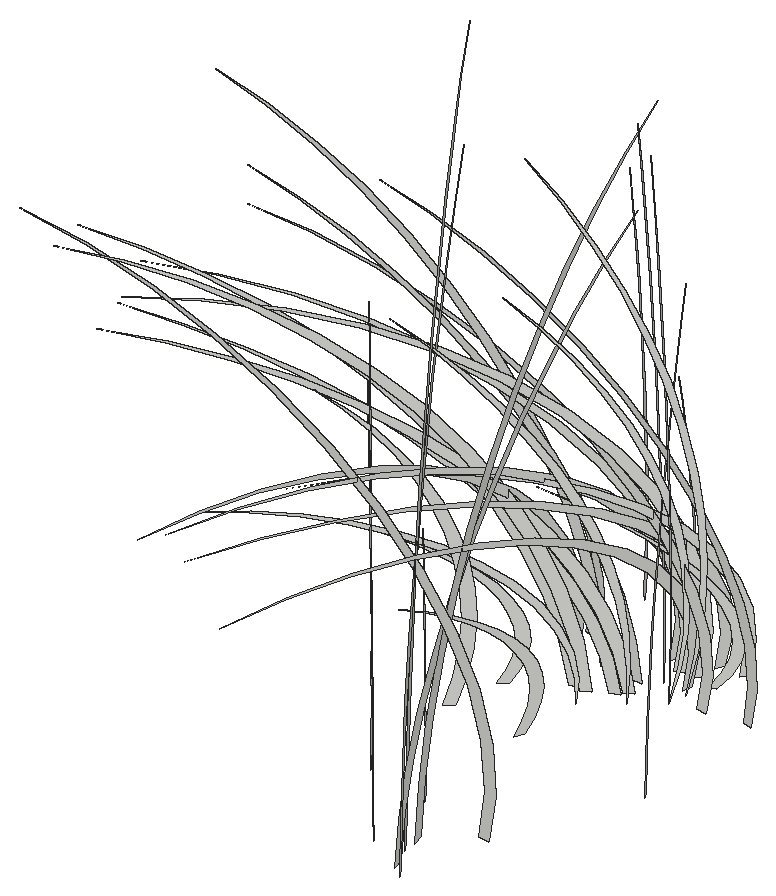
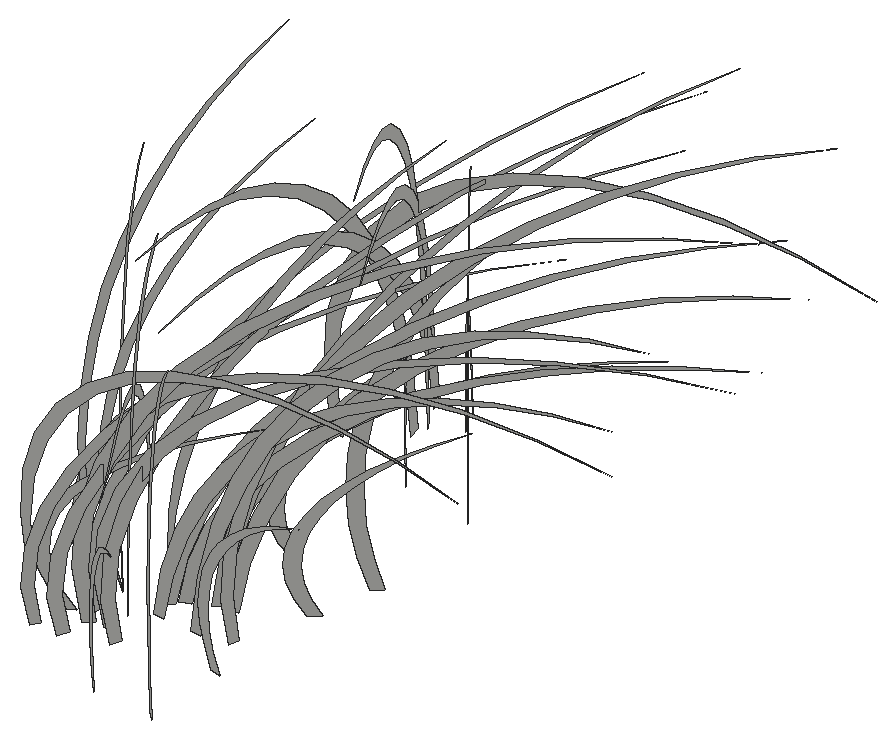
# SketchUp Ruby script. Lengths in inches.
U = 1.inch
M = Sketchup.active_model
def pt(a) = Geom::Point3d.new(a.map { |v| v * U })
def face(e, loops, mat)
  f = e.add_face(loops[0].map { |a| pt(a) })
  loops[1..].each { |l| e.add_face(l.map { |a| pt(a) }).erase! }
  f.material = f.back_material = mat if mat
  f
end
# faces: each face lists its corners as indices into pts; further lists are holes
def faces(e, pts, list, mat = nil) = list.each { |f| face(e, (f[0].is_a?(Array) ? f : [f]).map { |l| l.map { |i| pts[i] } }, mat) }
# xy, xz, yz: faces in a plane at the given z, y or x. An outline is a flat list of corners, or four numbers for a rectangle; further outlines are holes
def ring(l) = l.size == 4 ? [[l[0], l[1]], [l[2], l[1]], [l[2], l[3]], [l[0], l[3]]] : l.each_slice(2).to_a
def flat(e, list, mat, &to3) = list.each { |f| face(e, (f[0].is_a?(Array) ? f : [f]).map { |l| ring(l).map { |u, v| to3.(u, v) } }, mat) }
def xy(e, z, list, mat = nil) = flat(e, list, mat) { |x, y| [x, y, z] }
def xz(e, y, list, mat = nil) = flat(e, list, mat) { |x, z| [x, y, z] }
def yz(e, x, list, mat = nil) = flat(e, list, mat) { |y, z| [x, y, z] }
def lines(e, pts, list) = list.each { |a, b| e.add_line(pt(pts[a]), pt(pts[b])) }
# prism: a flat outline (further loops are holes) pulled along v
def prism(e, loops, v, mat = nil)
  f = face(e, loops, mat); d = Geom::Vector3d.new(v.map { |x| x * U })
  f.pushpull(f.normal.samedirection?(d) ? d.length : -d.length)
end
def box(e, o, s, mat = nil) = prism(e, [[o, [o[0] + s[0], o[1], o[2]], [o[0] + s[0], o[1] + s[1], o[2]], [o[0], o[1] + s[1], o[2]]]], [0, 0, s[2]], mat)
def at(x, y, z, deg = 0) = Geom::Transformation.translation(pt([x, y, z])) * Geom::Transformation.rotation(ORIGIN, Z_AXIS, deg.degrees)
def axes(o, x, y, z) = Geom::Transformation.new([*x, 0, *y, 0, *z, 0, *pt(o).to_a, 1])
def part(name) = M.definitions.add(name)
# library, detail: a bought-in or finely detailed component or shape, given as its bounding box
def library(name, o, s) = part(name).tap { |d| box(d.entities, o, s) }
def detail(e, o, s) = box(e.add_group.entities, o, s)
def put(e, d, t, mat = nil) = e.add_instance(d, t).tap { |i| i.material = mat if mat }
def group(e, t, mat = nil) = e.add_group.tap { |g| g.transformation = t; g.material = mat if mat }.entities
root = M.entities
g1 = group(root,at(60.56,581.97,0.02))
p = [[-17.05,1.34,17.08],[-19.62,1.54,17.53],[-17.13,1.35,16.98],[-14.72,1.16,16.23],[-12.43,0.98,15.27],[-10.27,0.81,14.125],
  [-8.28,0.65,12.8],[-6.47,0.51,11.3125],[-4.86,0.38,9.68],[-3.48,0.27,7.92],[-2.34,0.18,6.05],[-1.44,0.11,4.09],
  [-0.81,0.0625,2.07],[-0.44,0.03,0],[0,0,0],[-0.3,0.02,2.11],[-0.89,0.07,4.1875],[-1.77,0.14,6.19],
  [-2.92,0.23,8.11],[-4.34,0.34,9.9],[-5.99,0.47,11.56],[-7.86,0.62,13.05],[-9.93,0.78,14.37],[-12.17,0.96,15.49],
  [-14.55,1.15,16.39]]
faces(g1,p,[[0,1,2,3,4,5,6,7,8,9,10,11,12,13,14,15,16,17,18,19,20,21,22,23,24]])
g2 = group(root,at(60.53,580.25,0.02))
p = [[-16.35,-5,14.86],[-18.82,-5.75,15.25],[-16.43,-5.02,14.77],[-14.12,-4.32,14.12],[-11.92,-3.65,13.29],[-9.85,-3.01,12.29],
  [-7.94,-2.43,11.14],[-6.21,-1.9,9.84],[-4.67,-1.43,8.42],[-3.34,-1.02,6.89],[-2.24,-0.69,5.26],[-1.38,-0.42,3.56],
  [-0.78,-0.24,1.8],[-0.43,-0.13,0],[0,0,0],[-0.29,-0.09,1.84],[-0.86,-0.26,3.64],[-1.7,-0.52,5.39],
  [-2.81,-0.86,7.05],[-4.16,-1.27,8.62],[-5.75,-1.76,10.06],[-7.54,-2.31,11.36],[-9.53,-2.91,12.5],[-11.68,-3.57,13.47],
  [-13.96,-4.27,14.26]]
faces(g2,p,[[0,1,2,3,4,5,6,7,8,9,10,11,12,13,14,15,16,17,18,19,20,21,22,23,24]])
g3 = group(root,at(62.14,581.84,0.02))
p = [[-17.05,1.34,13.77],[-19.62,1.54,14.14],[-17.13,1.35,13.7],[-14.72,1.16,13.09],[-12.43,0.98,12.32],[-10.27,0.81,11.39],
  [-8.28,0.65,10.32],[-6.47,0.51,9.12],[-4.86,0.38,7.8],[-3.48,0.27,6.38],[-2.34,0.18,4.875],[-1.44,0.11,3.3],
  [-0.81,0.0625,1.67],[-0.44,0.03,0],[0,0,0],[-0.3,0.02,1.71],[-0.89,0.07,3.38],[-1.77,0.14,4.99],
  [-2.92,0.23,6.54],[-4.34,0.34,7.99],[-5.99,0.47,9.32],[-7.86,0.62,10.53],[-9.93,0.78,11.59],[-12.17,0.96,12.49],
  [-14.55,1.15,13.22]]
faces(g3,p,[[0,1,2,3,4,5,6,7,8,9,10,11,12,13,14,15,16,17,18,19,20,21,22,23,24]])
g4 = group(root,at(65.52,569.11,0.02))
p = [[-0.91,0.16,0],[-0.4,0.07,0],[0,0,2.0625],[-0.16,0.03,4.13],[-0.89,0.16,6.16],[-2.17,0.39,8.1],
  [-3.95,0.7,9.91],[-6.21,1.11,11.52],[-8.88,1.58,12.92],[-11.91,2.12,14.05],[-15.2,2.71,14.9],[-18.68,3.33,15.45],
  [-22.27,3.97,15.67],[-25.88,4.61,15.5625],[-22.34,3.98,15.58],[-18.84,3.36,15.29],[-15.45,2.75,14.71],[-12.26,2.18,13.83],
  [-9.34,1.66,12.68],[-6.75,1.2,11.3],[-4.56,0.8125,9.7],[-2.81,0.5,7.9375],[-1.55,0.28,6.04],[-0.8,0.14,4.05],
  [-0.59,0.1,2.02]]
faces(g4,p,[[0,1,2,3,4,5,6,7,8,9,10,11,12,13,14,15,16,17,18,19,20,21,22,23,24]])
g5 = group(root,at(65.52,569.11,0.02))
p = [[-0.91,0.16,0],[-0.4,0.07,0],[0,0,2.0625],[-0.16,0.03,4.13],[-0.89,0.16,6.16],[-2.17,0.39,8.1],
  [-3.95,0.7,9.91],[-6.21,1.11,11.52],[-8.88,1.58,12.92],[-11.91,2.12,14.05],[-15.2,2.71,14.9],[-18.68,3.33,15.45],
  [-22.27,3.97,15.67],[-25.88,4.61,15.5625],[-22.34,3.98,15.58],[-18.84,3.36,15.29],[-15.45,2.75,14.71],[-12.26,2.18,13.83],
  [-9.34,1.66,12.68],[-6.75,1.2,11.3],[-4.56,0.8125,9.7],[-2.81,0.5,7.9375],[-1.55,0.28,6.04],[-0.8,0.14,4.05],
  [-0.59,0.1,2.02]]
faces(g5,p,[[0,1,2,3,4,5,6,7,8,9,10,11,12,13,14,15,16,17,18,19,20,21,22,23,24]])
g6 = group(root,at(62.05,580.72,0.02))
p = [[-16.35,-5,11.98],[-18.82,-5.75,12.3],[-16.43,-5.02,11.91],[-14.12,-4.32,11.39],[-11.92,-3.65,10.71],[-9.85,-3.01,9.91],
  [-7.94,-2.43,8.98],[-6.21,-1.9,7.9375],[-4.67,-1.43,6.79],[-3.34,-1.02,5.55],[-2.24,-0.69,4.24],[-1.38,-0.42,2.87],
  [-0.78,-0.24,1.45],[-0.43,-0.13,0],[0,0,0],[-0.29,-0.09,1.48],[-0.86,-0.26,2.9375],[-1.7,-0.52,4.35],
  [-2.81,-0.86,5.6875],[-4.16,-1.27,6.95],[-5.75,-1.76,8.11],[-7.54,-2.31,9.16],[-9.53,-2.91,10.08],[-11.68,-3.57,10.87],
  [-13.96,-4.27,11.5]]
faces(g6,p,[[0,1,2,3,4,5,6,7,8,9,10,11,12,13,14,15,16,17,18,19,20,21,22,23,24]])
g7 = group(root,at(61.05,580.28,0.02))
p = [[-14.34,-9.3125,17.08],[-16.51,-10.72,17.53],[-14.41,-9.36,16.98],[-12.39,-8.04,16.23],[-10.46,-6.79,15.27],[-8.64,-5.61,14.125],
  [-6.96,-4.52,12.8],[-5.44,-3.53,11.3125],[-4.09,-2.66,9.68],[-2.93,-1.9,7.92],[-1.97,-1.28,6.05],[-1.21,-0.79,4.09],
  [-0.68,-0.44,2.07],[-0.375,-0.24,0],[0,0,0],[-0.25,-0.16,2.11],[-0.75,-0.49,4.1875],[-1.49,-0.97,6.19],
  [-2.46,-1.6,8.11],[-3.65,-2.37,9.9],[-5.04,-3.27,11.56],[-6.61,-4.3,13.05],[-8.36,-5.43,14.37],[-10.24,-6.65,15.49],
  [-12.24,-7.95,16.39]]
faces(g7,p,[[0,1,2,3,4,5,6,7,8,9,10,11,12,13,14,15,16,17,18,19,20,21,22,23,24]])
g8 = group(root,at(63.18,583.56,0.02))
p = [[-0.73,-0.22,0],[-0.32,-0.1,0],[0,0,1.7],[-0.13,-0.04,3.4],[-0.71,-0.22,5.07],[-1.73,-0.53,6.67],
  [-3.16,-0.97,8.15],[-4.97,-1.52,9.48],[-7.1,-2.17,10.63],[-9.52,-2.91,11.57],[-12.15,-3.71,12.27],[-14.9375,-4.57,12.71],
  [-17.81,-5.44,12.89],[-20.6875,-6.33,12.81],[-17.86,-5.46,12.82],[-15.0625,-4.6,12.59],[-12.35,-3.78,12.1],[-9.8,-3,11.38],
  [-7.47,-2.28,10.4375],[-5.4,-1.65,9.3],[-3.64,-1.11,7.99],[-2.25,-0.6875,6.53],[-1.24,-0.38,4.97],[-0.64,-0.2,3.33],
  [-0.47,-0.14,1.67]]
faces(g8,p,[[0,1,2,3,4,5,6,7,8,9,10,11,12,13,14,15,16,17,18,19,20,21,22,23,24]])
g9 = group(root,at(65.68,581.57,0.02))
p = [[-0.81,0.0625,0],[-0.36,0.03,0],[0,0,1.66],[-0.15,0.01,3.32],[-0.8,0.0625,4.96],[-1.9375,0.15,6.52],
  [-3.54,0.28,7.97],[-5.56,0.4375,9.27],[-7.95,0.625,10.39],[-10.65,0.84,11.3],[-13.6,1.07,11.98],[-16.72,1.32,12.42],
  [-19.93,1.57,12.6],[-23.15,1.82,12.51],[-19.99,1.57,12.53],[-16.85,1.33,12.3],[-13.83,1.09,11.82],[-10.97,0.86,11.12],
  [-8.35,0.66,10.2],[-6.04,0.48,9.09],[-4.08,0.32,7.8],[-2.51,0.2,6.38],[-1.39,0.11,4.86],[-0.72,0.06,3.26],
  [-0.53,0.04,1.63]]
faces(g9,p,[[0,1,2,3,4,5,6,7,8,9,10,11,12,13,14,15,16,17,18,19,20,21,22,23,24]])
g10 = group(root,at(62.38,581.15,0.02))
p = [[-14.34,-9.3125,13.77],[-16.51,-10.72,14.14],[-14.41,-9.36,13.7],[-12.39,-8.04,13.09],[-10.46,-6.79,12.32],[-8.64,-5.61,11.39],
  [-6.96,-4.52,10.32],[-5.44,-3.53,9.12],[-4.09,-2.66,7.8],[-2.93,-1.9,6.38],[-1.97,-1.28,4.875],[-1.21,-0.79,3.3],
  [-0.68,-0.44,1.67],[-0.375,-0.24,0],[0,0,0],[-0.25,-0.16,1.71],[-0.75,-0.49,3.38],[-1.49,-0.97,4.99],
  [-2.46,-1.6,6.54],[-3.65,-2.37,7.99],[-5.04,-3.27,9.32],[-6.61,-4.3,10.53],[-8.36,-5.43,11.59],[-10.24,-6.65,12.49],
  [-12.24,-7.95,13.22]]
faces(g10,p,[[0,1,2,3,4,5,6,7,8,9,10,11,12,13,14,15,16,17,18,19,20,21,22,23,24]])
g11 = group(root,at(63.88,583.79,0.02))
p = [[-0.64,-0.41,0],[-0.28,-0.18,0],[0,0,1.95],[-0.11,-0.07,3.91],[-0.625,-0.41,5.83],[-1.52,-0.99,7.67],
  [-2.77,-1.8,9.37],[-4.36,-2.83,10.9],[-6.23,-4.05,12.22],[-8.35,-5.42,13.3],[-10.66,-6.92,14.1],[-13.1,-8.51,14.61],
  [-15.62,-10.14,14.82],[-18.14,-11.78,14.72],[-15.66,-10.17,14.74],[-13.21,-8.58,14.47],[-10.83,-7.04,13.91],[-8.6,-5.58,13.08],
  [-6.55,-4.25,12],[-4.73,-3.07,10.6875],[-3.19,-2.07,9.18],[-1.97,-1.28,7.51],[-1.09,-0.7,5.71],[-0.5625,-0.37,3.83],
  [-0.41,-0.27,1.91]]
faces(g11,p,[[0,1,2,3,4,5,6,7,8,9,10,11,12,13,14,15,16,17,18,19,20,21,22,23,24]])
g12 = group(root,at(61.27,579.25,0.02))
p = [[-10.68,-8.77,8.14],[-9.25,-7.59,8.09],[-7.83,-6.43,7.89],[-6.47,-5.32,7.56],[-5.19,-4.26,7.08],[-4,-3.29,6.49],
  [-2.94,-2.42,5.78],[-2.02,-1.66,4.97],[-1.27,-1.04,4.07],[-0.6875,-0.56,3.11],[-0.29,-0.24,2.09],[-0.1,-0.08,1.05],
  [-0.09,-0.08,0],[0,0,1.07],[-0.125,-0.1,2.14],[-0.47,-0.38,3.19],[-1.02,-0.84,4.1875],[-1.77,-1.45,5.11],
  [-2.7,-2.22,5.94],[-3.79,-3.11,6.67],[-5.01,-4.12,7.26],[-6.35,-5.21,7.71],[-7.76,-6.37,8.02],[-9.21,-7.57,8.16]]
faces(g12,p,[[0,1,2,3,4,5,6,7,8,9,10,11,12,13,14,15,16,17,18,19,20,21,22,23]])
g13 = group(root,at(58.4,576.89,0.02))
p = [[-4.57,-3.75,13.1875],[-3.73,-3.06,12.35],[-2.98,-2.45,11.43],[-2.3125,-1.9,10.45],[-1.74,-1.43,9.4],[-1.26,-1.04,8.29],
  [-0.89,-0.73,7.15],[-0.63,-0.52,5.97],[-0.47,-0.39,4.78],[-0.43,-0.35,3.57],[-0.49,-0.41,2.36],[-0.67,-0.55,1.17],
  [-0.96,-0.78,0],[-0.59,-0.48,0],[-0.27,-0.22,1.1875],[-0.07,-0.0625,2.4],[0,0,3.63],[-0.05,-0.04,4.86],
  [-0.22,-0.18,6.08],[-0.52,-0.43,7.27],[-0.93,-0.76,8.42],[-1.46,-1.2,9.52],[-2.09,-1.72,10.5625],[-2.83,-2.32,11.53],
  [-3.65,-3,12.41]]
faces(g13,p,[[0,1,2,3,4,5,6,7,8,9,10,11,12,13,14,15,16,17,18,19,20,21,22,23,24]])
g14 = group(root,at(58.4,576.89,0.02))
p = [[-4.57,-3.75,13.1875],[-3.73,-3.06,12.35],[-2.98,-2.45,11.43],[-2.3125,-1.9,10.45],[-1.74,-1.43,9.4],[-1.26,-1.04,8.29],
  [-0.89,-0.73,7.15],[-0.63,-0.52,5.97],[-0.47,-0.39,4.78],[-0.43,-0.35,3.57],[-0.49,-0.41,2.36],[-0.67,-0.55,1.17],
  [-0.96,-0.78,0],[-0.59,-0.48,0],[-0.27,-0.22,1.1875],[-0.07,-0.0625,2.4],[0,0,3.63],[-0.05,-0.04,4.86],
  [-0.22,-0.18,6.08],[-0.52,-0.43,7.27],[-0.93,-0.76,8.42],[-1.46,-1.2,9.52],[-2.09,-1.72,10.5625],[-2.83,-2.32,11.53],
  [-3.65,-3,12.41]]
faces(g14,p,[[0,1,2,3,4,5,6,7,8,9,10,11,12,13,14,15,16,17,18,19,20,21,22,23,24]])
g15 = group(root,at(67.6,581.72,0.02))
p = [[-0.79,0.21,0],[-0.35,0.09,0],[0,0,1.66],[-0.14,0.04,3.32],[-0.77,0.21,4.96],[-1.875,0.51,6.52],
  [-3.43,0.92,7.97],[-5.38,1.45,9.27],[-7.7,2.08,10.39],[-10.32,2.78,11.3],[-13.17,3.55,11.98],[-16.1875,4.37,12.42],
  [-19.3,5.21,12.6],[-22.42,6.05,12.51],[-19.36,5.22,12.53],[-16.32,4.4,12.3],[-13.39,3.61,11.82],[-10.625,2.87,11.12],
  [-8.09,2.18,10.2],[-5.85,1.58,9.09],[-3.95,1.07,7.8],[-2.43,0.66,6.38],[-1.34,0.36,4.86],[-0.69,0.1875,3.26],
  [-0.51,0.14,1.63]]
faces(g15,p,[[0,1,2,3,4,5,6,7,8,9,10,11,12,13,14,15,16,17,18,19,20,21,22,23,24]])
g16 = group(root,at(59.24,583.24,0.02))
p = [[-5.59,1.92,7.46],[-4.57,1.57,6.98],[-3.64,1.25,6.46],[-2.83,0.97,5.91],[-2.125,0.73,5.3125],[-1.55,0.53,4.6875],
  [-1.09,0.375,4.04],[-0.77,0.26,3.38],[-0.58,0.2,2.7],[-0.52,0.18,2.02],[-0.61,0.21,1.34],[-0.82,0.28,0.66],
  [-1.17,0.4,0],[-0.72,0.25,0],[-0.33,0.11,0.67],[-0.09,0.03,1.36],[0,0,2.05],[-0.0625,0.02,2.75],
  [-0.27,0.09,3.4375],[-0.63,0.22,4.11],[-1.14,0.39,4.76],[-1.78,0.61,5.39],[-2.56,0.88,5.97],[-3.46,1.19,6.52],
  [-4.47,1.54,7.01]]
faces(g16,p,[[0,1,2,3,4,5,6,7,8,9,10,11,12,13,14,15,16,17,18,19,20,21,22,23,24]])
g17 = group(root,at(61.87,566.53,0.02))
p = [[-10.66,12.98,9.9],[-9.23,11.23,9.83],[-7.82,9.52,9.59],[-6.46,7.86,9.18],[-5.18,6.3,8.61],[-3.99,4.86,7.88],
  [-2.93,3.57,7.02],[-2.02,2.46,6.03],[-1.27,1.54,4.95],[-0.6875,0.84,3.78],[-0.29,0.36,2.55],[-0.1,0.12,1.28],
  [-0.09,0.12,0],[0,0,1.3],[-0.125,0.15,2.61],[-0.47,0.57,3.875],[-1.02,1.24,5.09],[-1.77,2.15,6.21],
  [-2.69,3.28,7.22],[-3.78,4.6,8.1],[-5,6.09,8.82],[-6.33,7.71,9.37],[-7.74,9.43,9.74],[-9.2,11.19,9.92]]
faces(g17,p,[[0,1,2,3,4,5,6,7,8,9,10,11,12,13,14,15,16,17,18,19,20,21,22,23]])
g18 = group(root,at(63.12,566.8,0.02))
p = [[-11.32,17.43,20.75],[-13.02,20.05,21.3],[-11.37,17.51,20.63],[-9.77,15.05,19.72],[-8.25,12.7,18.55],[-6.82,10.5,17.16],
  [-5.5,8.46,15.55],[-4.29,6.61,13.74],[-3.23,4.97,11.76],[-2.3125,3.56,9.62],[-1.55,2.39,7.35],[-0.96,1.47,4.97],
  [-0.54,0.83,2.51],[-0.29,0.45,0],[0,0,0],[-0.2,0.31,2.57],[-0.59,0.91,5.09],[-1.18,1.8125,7.53],
  [-1.94,2.99,9.85],[-2.88,4.43,12.03],[-3.98,6.12,14.04],[-5.22,8.04,15.86],[-6.59,10.15,17.46],[-8.08,12.44,18.82],
  [-9.66,14.88,19.92]]
faces(g18,p,[[0,1,2,3,4,5,6,7,8,9,10,11,12,13,14,15,16,17,18,19,20,21,22,23,24]])
g19 = group(root,at(58.93,579.38,0.02))
p = [[-4.57,-3.75,6.49],[-3.73,-3.06,6.08],[-2.98,-2.45,5.625],[-2.3125,-1.9,5.14],[-1.74,-1.43,4.62],[-1.26,-1.04,4.08],
  [-0.89,-0.73,3.52],[-0.63,-0.52,2.9375],[-0.47,-0.39,2.35],[-0.43,-0.35,1.76],[-0.49,-0.41,1.16],[-0.67,-0.55,0.58],
  [-0.96,-0.78,0],[-0.59,-0.48,0],[-0.27,-0.22,0.58],[-0.07,-0.0625,1.18],[0,0,1.78],[-0.05,-0.04,2.39],
  [-0.22,-0.18,2.99],[-0.52,-0.43,3.58],[-0.93,-0.76,4.14],[-1.46,-1.2,4.69],[-2.09,-1.72,5.2],[-2.83,-2.32,5.67],
  [-3.65,-3,6.1]]
faces(g19,p,[[0,1,2,3,4,5,6,7,8,9,10,11,12,13,14,15,16,17,18,19,20,21,22,23,24]])
g20 = group(root,at(59,570.02,0.02))
p = [[-4.56,5.55,16.02],[-3.72,4.53,15.01],[-2.97,3.62,13.89],[-2.31,2.81,12.69],[-1.73,2.11,11.42],[-1.26,1.54,10.08],
  [-0.89,1.09,8.6875],[-0.63,0.76,7.26],[-0.47,0.58,5.8],[-0.43,0.52,4.34],[-0.49,0.6,2.87],[-0.67,0.81,1.42],
  [-0.95,1.16,0],[-0.59,0.71,0],[-0.27,0.33,1.44],[-0.07,0.09,2.92],[0,0,4.41],[-0.05,0.0625,5.9],
  [-0.22,0.27,7.38],[-0.52,0.63,8.83],[-0.93,1.13,10.23],[-1.45,1.77,11.57],[-2.09,2.54,12.83],[-2.82,3.43,14.01],
  [-3.65,4.44,15.07]]
faces(g20,p,[[0,1,2,3,4,5,6,7,8,9,10,11,12,13,14,15,16,17,18,19,20,21,22,23,24]])
g21 = group(root,at(59,570.02,0.02))
p = [[-4.56,5.55,16.02],[-3.72,4.53,15.01],[-2.97,3.62,13.89],[-2.31,2.81,12.69],[-1.73,2.11,11.42],[-1.26,1.54,10.08],
  [-0.89,1.09,8.6875],[-0.63,0.76,7.26],[-0.47,0.58,5.8],[-0.43,0.52,4.34],[-0.49,0.6,2.87],[-0.67,0.81,1.42],
  [-0.95,1.16,0],[-0.59,0.71,0],[-0.27,0.33,1.44],[-0.07,0.09,2.92],[0,0,4.41],[-0.05,0.0625,5.9],
  [-0.22,0.27,7.38],[-0.52,0.63,8.83],[-0.93,1.13,10.23],[-1.45,1.77,11.57],[-2.09,2.54,12.83],[-2.82,3.43,14.01],
  [-3.65,4.44,15.07]]
faces(g21,p,[[0,1,2,3,4,5,6,7,8,9,10,11,12,13,14,15,16,17,18,19,20,21,22,23,24]])
g22 = group(root,at(58.86,586.28,0.02))
p = [[-4.18,4.18,15.16],[-3.41,3.41,14.2],[-2.72,2.72,13.14],[-2.11,2.11,12.01],[-1.59,1.59,10.8],[-1.16,1.16,9.53],
  [-0.82,0.82,8.22],[-0.58,0.58,6.87],[-0.43,0.43,5.49],[-0.39,0.39,4.1],[-0.45,0.45,2.72],[-0.61,0.61,1.35],
  [-0.875,0.875,0],[-0.54,0.54,0],[-0.25,0.25,1.36],[-0.07,0.07,2.76],[0,0,4.17],[-0.05,0.05,5.58],
  [-0.2,0.2,6.98],[-0.47,0.47,8.35],[-0.85,0.85,9.68],[-1.33,1.33,10.95],[-1.91,1.91,12.14],[-2.59,2.59,13.25],
  [-3.34,3.34,14.26]]
faces(g22,p,[[0,1,2,3,4,5,6,7,8,9,10,11,12,13,14,15,16,17,18,19,20,21,22,23,24]])
g23 = group(root,at(59.14,582.25,0.02))
p = [[-0.13,-0.75,0],[-0.06,-0.33,0],[0,0,1.7],[-0.02,-0.13,3.4],[-0.13,-0.73,5.07],[-0.32,-1.78,6.67],
  [-0.58,-3.25,8.15],[-0.91,-5.11,9.48],[-1.3,-7.3125,10.63],[-1.75,-9.8,11.57],[-2.23,-12.51,12.27],[-2.74,-15.375,12.71],
  [-3.27,-18.33,12.89],[-3.79,-21.3,12.81],[-3.28,-18.39,12.82],[-2.76,-15.5,12.59],[-2.27,-12.72,12.1],[-1.8,-10.09,11.38],
  [-1.37,-7.69,10.4375],[-0.99,-5.56,9.3],[-0.67,-3.75,7.99],[-0.41,-2.3125,6.53],[-0.23,-1.27,4.97],[-0.12,-0.66,3.33],
  [-0.09,-0.48,1.67]]
faces(g23,p,[[0,1,2,3,4,5,6,7,8,9,10,11,12,13,14,15,16,17,18,19,20,21,22,23,24]])
g24 = group(root,at(59.14,582.25,0.02))
p = [[-0.13,-0.75,0],[-0.06,-0.33,0],[0,0,1.7],[-0.02,-0.13,3.4],[-0.13,-0.73,5.07],[-0.32,-1.78,6.67],
  [-0.58,-3.25,8.15],[-0.91,-5.11,9.48],[-1.3,-7.3125,10.63],[-1.75,-9.8,11.57],[-2.23,-12.51,12.27],[-2.74,-15.375,12.71],
  [-3.27,-18.33,12.89],[-3.79,-21.3,12.81],[-3.28,-18.39,12.82],[-2.76,-15.5,12.59],[-2.27,-12.72,12.1],[-1.8,-10.09,11.38],
  [-1.37,-7.69,10.4375],[-0.99,-5.56,9.3],[-0.67,-3.75,7.99],[-0.41,-2.3125,6.53],[-0.23,-1.27,4.97],[-0.12,-0.66,3.33],
  [-0.09,-0.48,1.67]]
faces(g24,p,[[0,1,2,3,4,5,6,7,8,9,10,11,12,13,14,15,16,17,18,19,20,21,22,23,24]])
g25 = group(root,at(64.17,565.18,0.02))
p = [[-11.32,17.43,16.73],[-13.02,20.05,17.17],[-11.37,17.51,16.64],[-9.77,15.05,15.9],[-8.25,12.7,14.96],[-6.82,10.5,13.84],
  [-5.5,8.46,12.54],[-4.29,6.61,11.08],[-3.23,4.97,9.48],[-2.3125,3.56,7.76],[-1.55,2.39,5.92],[-0.96,1.47,4.01],
  [-0.54,0.83,2.02],[-0.29,0.45,0],[0,0,0],[-0.2,0.31,2.07],[-0.59,0.91,4.1],[-1.18,1.8125,6.07],
  [-1.94,2.99,7.94],[-2.88,4.43,9.7],[-3.98,6.12,11.33],[-5.22,8.04,12.79],[-6.59,10.15,14.08],[-8.08,12.44,15.17],
  [-9.66,14.88,16.0625]]
faces(g25,p,[[0,1,2,3,4,5,6,7,8,9,10,11,12,13,14,15,16,17,18,19,20,21,22,23,24]])
g26 = group(root,at(62.08,584.6,0.02))
p = [[-0.23,-0.78,0],[-0.1,-0.35,0],[0,0,1.66],[-0.04,-0.14,3.32],[-0.22,-0.77,4.96],[-0.55,-1.87,6.52],
  [-1,-3.41,7.97],[-1.56,-5.35,9.27],[-2.24,-7.65,10.39],[-3,-10.25,11.3],[-3.83,-13.09,11.98],[-4.71,-16.09,12.42],
  [-5.61,-19.19,12.6],[-6.52,-22.29,12.51],[-5.63,-19.24,12.53],[-4.75,-16.23,12.3],[-3.89,-13.3125,11.82],[-3.09,-10.5625,11.12],
  [-2.35,-8.04,10.2],[-1.7,-5.8125,9.09],[-1.15,-3.93,7.8],[-0.71,-2.42,6.38],[-0.39,-1.33,4.86],[-0.2,-0.69,3.26],
  [-0.15,-0.51,1.63]]
faces(g26,p,[[0,1,2,3,4,5,6,7,8,9,10,11,12,13,14,15,16,17,18,19,20,21,22,23,24]])
g27 = group(root,at(61.39,586,0.02))
p = [[-4.18,4.18,7.46],[-3.41,3.41,6.98],[-2.72,2.72,6.46],[-2.11,2.11,5.91],[-1.59,1.59,5.3125],[-1.16,1.16,4.6875],
  [-0.82,0.82,4.04],[-0.58,0.58,3.38],[-0.43,0.43,2.7],[-0.39,0.39,2.02],[-0.45,0.45,1.34],[-0.61,0.61,0.66],
  [-0.875,0.875,0],[-0.54,0.54,0],[-0.25,0.25,0.67],[-0.07,0.07,1.36],[0,0,2.05],[-0.05,0.05,2.75],
  [-0.2,0.2,3.4375],[-0.47,0.47,4.11],[-0.85,0.85,4.76],[-1.33,1.33,5.39],[-1.91,1.91,5.97],[-2.59,2.59,6.52],
  [-3.34,3.34,7.01]]
faces(g27,p,[[0,1,2,3,4,5,6,7,8,9,10,11,12,13,14,15,16,17,18,19,20,21,22,23,24]])
g28 = group(root,at(62.72,580.4375,0.02))
p = [[-6.75,-5.55,16.14],[-5.68,-4.66,14.95],[-4.6875,-3.85,13.72],[-3.79,-3.11,12.45],[-2.98,-2.45,11.15],[-2.27,-1.87,9.82],
  [-1.66,-1.36,8.46],[-1.14,-0.9375,7.08],[-0.73,-0.6,5.6875],[-0.41,-0.34,4.28],[-0.2,-0.17,2.86],[-0.09,-0.08,1.43],
  [-0.09,-0.07,0],[0,0,1.4375],[-0.03,-0.03,2.875],[-0.1875,-0.15,4.31],[-0.46,-0.38,5.73],[-0.85,-0.7,7.14],
  [-1.36,-1.12,8.53],[-1.99,-1.63,9.89],[-2.73,-2.24,11.22],[-3.58,-2.9375,12.52],[-4.53,-3.72,13.77],[-5.59,-4.59,14.98]]
faces(g28,p,[[0,1,2,3,4,5,6,7,8,9,10,11,12,13,14,15,16,17,18,19,20,21,22,23]])
g29 = group(root,at(62.72,580.4375,0.02))
p = [[-6.75,-5.55,16.14],[-5.68,-4.66,14.95],[-4.6875,-3.85,13.72],[-3.79,-3.11,12.45],[-2.98,-2.45,11.15],[-2.27,-1.87,9.82],
  [-1.66,-1.36,8.46],[-1.14,-0.9375,7.08],[-0.73,-0.6,5.6875],[-0.41,-0.34,4.28],[-0.2,-0.17,2.86],[-0.09,-0.08,1.43],
  [-0.09,-0.07,0],[0,0,1.4375],[-0.03,-0.03,2.875],[-0.1875,-0.15,4.31],[-0.46,-0.38,5.73],[-0.85,-0.7,7.14],
  [-1.36,-1.12,8.53],[-1.99,-1.63,9.89],[-2.73,-2.24,11.22],[-3.58,-2.9375,12.52],[-4.53,-3.72,13.77],[-5.59,-4.59,14.98]]
faces(g29,p,[[0,1,2,3,4,5,6,7,8,9,10,11,12,13,14,15,16,17,18,19,20,21,22,23]])
g30 = group(root,at(63.09,567.43,0.02))
p = [[-6.07,19.87,18.05],[-6.99,22.87,18.53],[-6.1,19.96,17.95],[-5.25,17.16,17.15],[-4.43,14.49,16.14],[-3.66,11.97,14.93],
  [-2.95,9.65,13.53],[-2.31,7.54,11.96],[-1.73,5.67,10.23],[-1.24,4.06,8.37],[-0.83,2.72,6.39],[-0.51,1.68,4.32],
  [-0.29,0.94,2.18],[-0.16,0.52,0],[0,0,0],[-0.11,0.35,2.23],[-0.32,1.04,4.43],[-0.63,2.07,6.55],
  [-1.04,3.41,8.57],[-1.55,5.05,10.47],[-2.13,6.98,12.22],[-2.8,9.16,13.8],[-3.54,11.58,15.1875],[-4.34,14.1875,16.37],
  [-5.1875,16.96,17.33]]
faces(g30,p,[[0,1,2,3,4,5,6,7,8,9,10,11,12,13,14,15,16,17,18,19,20,21,22,23,24]])
g31 = group(root,at(63.79,585.14,0.02))
p = [[-0.29,-0.76,0],[-0.13,-0.34,0],[0,0,1.44],[-0.05,-0.14,2.89],[-0.28,-0.75,4.3125],[-0.6875,-1.82,5.67],
  [-1.25,-3.32,6.93],[-1.97,-5.21,8.0625],[-2.82,-7.46,9.04],[-3.78,-9.99,9.83],[-4.82,-12.76,10.43],[-5.93,-15.68,10.81],
  [-7.07,-18.7,10.96],[-8.21,-21.73,10.89],[-7.09,-18.76,10.9],[-5.98,-15.82,10.7],[-4.9,-12.97,10.29],[-3.89,-10.29,9.67],
  [-2.96,-7.84,8.875],[-2.14,-5.67,7.9],[-1.45,-3.83,6.79],[-0.89,-2.36,5.55],[-0.49,-1.3,4.22],[-0.25,-0.67,2.83],
  [-0.1875,-0.49,1.42]]
faces(g31,p,[[0,1,2,3,4,5,6,7,8,9,10,11,12,13,14,15,16,17,18,19,20,21,22,23,24]])
g32 = group(root,at(62.81,582.33,0.02))
p = [[-6.18,6.18,18.55],[-5.19,5.19,17.18],[-4.29,4.29,15.77],[-3.47,3.47,14.31],[-2.73,2.73,12.8125],[-2.08,2.08,11.28],
  [-1.52,1.52,9.73],[-1.04,1.04,8.14],[-0.66,0.66,6.54],[-0.38,0.38,4.91],[-0.18,0.18,3.28],[-0.09,0.09,1.64],
  [-0.08,0.08,0],[0,0,1.65],[-0.03,0.03,3.3],[-0.17,0.17,4.95],[-0.42,0.42,6.59],[-0.78,0.78,8.2],
  [-1.25,1.25,9.8],[-1.82,1.82,11.37],[-2.5,2.5,12.9],[-3.27,3.27,14.39],[-4.15,4.15,15.83],[-5.12,5.12,17.22]]
faces(g32,p,[[0,1,2,3,4,5,6,7,8,9,10,11,12,13,14,15,16,17,18,19,20,21,22,23]])
g33 = group(root,at(62.03,569.38,0.02))
p = [[-4.56,5.55,7.88],[-3.72,4.53,7.38],[-2.97,3.62,6.83],[-2.31,2.81,6.24],[-1.73,2.11,5.62],[-1.26,1.54,4.96],
  [-0.89,1.09,4.27],[-0.63,0.76,3.57],[-0.47,0.58,2.86],[-0.43,0.52,2.13],[-0.49,0.6,1.41],[-0.67,0.81,0.7],
  [-0.95,1.16,0],[-0.59,0.71,0],[-0.27,0.33,0.71],[-0.07,0.09,1.43],[0,0,2.17],[-0.05,0.0625,2.9],
  [-0.22,0.27,3.63],[-0.52,0.63,4.34],[-0.93,1.13,5.03],[-1.45,1.77,5.69],[-2.09,2.54,6.3125],[-2.82,3.43,6.89],
  [-3.65,4.44,7.41]]
faces(g33,p,[[0,1,2,3,4,5,6,7,8,9,10,11,12,13,14,15,16,17,18,19,20,21,22,23,24]])
g34 = group(root,at(64.93,585.01,0.02))
p = [[-0.36,-0.51,0],[-0.16,-0.23,0],[0,0,1.38],[-0.07,-0.09,2.78],[-0.36,-0.5,4.14],[-0.87,-1.21,5.44],
  [-1.58,-2.2,6.65],[-2.48,-3.46,7.74],[-3.55,-4.95,8.68],[-4.76,-6.63,9.44],[-6.08,-8.46,10.01],[-7.47,-10.4,10.375],
  [-8.91,-12.4,10.52],[-10.35,-14.41,10.45],[-8.9375,-12.4375,10.47],[-7.54,-10.49,10.27],[-6.18,-8.6,9.88],[-4.9,-6.83,9.29],
  [-3.74,-5.2,8.52],[-2.7,-3.76,7.59],[-1.82,-2.54,6.52],[-1.125,-1.5625,5.33],[-0.62,-0.86,4.06],[-0.32,-0.45,2.72],
  [-0.24,-0.33,1.36]]
faces(g34,p,[[0,1,2,3,4,5,6,7,8,9,10,11,12,13,14,15,16,17,18,19,20,21,22,23,24]])
g35 = group(root,at(63.65,565.59,0.02))
p = [[-6.07,19.87,14.56],[-6.99,22.87,14.94],[-6.1,19.96,14.48],[-5.25,17.16,13.83],[-4.43,14.49,13.02],[-3.66,11.97,12.04],
  [-2.95,9.65,10.91],[-2.31,7.54,9.64],[-1.73,5.67,8.25],[-1.24,4.06,6.75],[-0.83,2.72,5.15],[-0.51,1.68,3.49],
  [-0.29,0.94,1.76],[-0.16,0.52,0],[0,0,0],[-0.11,0.35,1.8],[-0.32,1.04,3.57],[-0.63,2.07,5.28],
  [-1.04,3.41,6.91],[-1.55,5.05,8.44],[-2.13,6.98,9.85],[-2.8,9.16,11.13],[-3.54,11.58,12.25],[-4.34,14.1875,13.2],
  [-5.1875,16.96,13.97]]
faces(g35,p,[[0,1,2,3,4,5,6,7,8,9,10,11,12,13,14,15,16,17,18,19,20,21,22,23,24]])
g36 = group(root,at(61.46,576.97,0.02))
p = [[-2.46,-5.37,6.49],[-2.01,-4.39,6.08],[-1.6,-3.5,5.625],[-1.24,-2.72,5.14],[-0.9375,-2.04,4.62],[-0.68,-1.49,4.08],
  [-0.48,-1.05,3.52],[-0.34,-0.74,2.9375],[-0.26,-0.56,2.35],[-0.23,-0.5,1.76],[-0.27,-0.58,1.16],[-0.36,-0.79,0.58],
  [-0.51,-1.125,0],[-0.32,-0.69,0],[-0.15,-0.32,0.58],[-0.04,-0.09,1.18],[0,0,1.78],[-0.03,-0.06,2.39],
  [-0.12,-0.26,2.99],[-0.28,-0.61,3.58],[-0.5,-1.1,4.14],[-0.79,-1.71,4.69],[-1.125,-2.46,5.2],[-1.52,-3.33,5.67],
  [-1.97,-4.3,6.1]]
faces(g36,p,[[0,1,2,3,4,5,6,7,8,9,10,11,12,13,14,15,16,17,18,19,20,21,22,23,24]])
g37 = group(root,at(64.66,582.49,0.02))
p = [[-0.71,-0.33,0],[-0.32,-0.15,1.86],[-0.08,-0.04,3.74],[0,0,5.63],[-0.08,-0.04,7.52],[-0.3125,-0.15,9.4],
  [-0.7,-0.33,11.26],[-1.24,-0.58,13.1],[-1.9375,-0.91,14.91],[-2.78,-1.3,16.68],[-3.77,-1.77,18.39],[-4.9,-2.29,20.06],
  [-6.16,-2.89,21.66],[-4.97,-2.33,20.03],[-3.91,-1.83,18.35],[-2.97,-1.39,16.625],[-2.17,-1.01,14.86],[-1.5,-0.7,13.05],
  [-0.96,-0.45,11.22],[-0.57,-0.27,9.37],[-0.3125,-0.15,7.5],[-0.2,-0.09,5.62],[-0.23,-0.11,3.74],[-0.4,-0.1875,1.86]]
faces(g37,p,[[0,1,2,3,4,5,6,7,8,9,10,11,12,13,14,15,16,17,18,19,20,21,22,23]])
g38 = group(root,at(63.75,583.21,0.02))
p = [[-0.14,-0.8,0],[-0.0625,-0.36,0],[0,0,1.44],[-0.03,-0.14,2.89],[-0.14,-0.79,4.3125],[-0.34,-1.91,5.67],
  [-0.62,-3.49,6.93],[-0.98,-5.49,8.0625],[-1.4,-7.85,9.04],[-1.875,-10.52,9.83],[-2.39,-13.43,10.43],[-2.94,-16.51,10.81],
  [-3.51,-19.68,10.96],[-4.07,-22.86,10.89],[-3.52,-19.74,10.9],[-2.96,-16.64,10.7],[-2.43,-13.65,10.29],[-1.93,-10.83,9.67],
  [-1.47,-8.25,8.875],[-1.0625,-5.96,7.9],[-0.72,-4.03,6.79],[-0.44,-2.48,5.55],[-0.24,-1.37,4.22],[-0.125,-0.71,2.83],
  [-0.09,-0.52,1.42]]
faces(g38,p,[[0,1,2,3,4,5,6,7,8,9,10,11,12,13,14,15,16,17,18,19,20,21,22,23,24]])
g39 = group(root,at(63.75,583.21,0.02))
p = [[-0.14,-0.8,0],[-0.0625,-0.36,0],[0,0,1.44],[-0.03,-0.14,2.89],[-0.14,-0.79,4.3125],[-0.34,-1.91,5.67],
  [-0.62,-3.49,6.93],[-0.98,-5.49,8.0625],[-1.4,-7.85,9.04],[-1.875,-10.52,9.83],[-2.39,-13.43,10.43],[-2.94,-16.51,10.81],
  [-3.51,-19.68,10.96],[-4.07,-22.86,10.89],[-3.52,-19.74,10.9],[-2.96,-16.64,10.7],[-2.43,-13.65,10.29],[-1.93,-10.83,9.67],
  [-1.47,-8.25,8.875],[-1.0625,-5.96,7.9],[-0.72,-4.03,6.79],[-0.44,-2.48,5.55],[-0.24,-1.37,4.22],[-0.125,-0.71,2.83],
  [-0.09,-0.52,1.42]]
faces(g39,p,[[0,1,2,3,4,5,6,7,8,9,10,11,12,13,14,15,16,17,18,19,20,21,22,23,24]])
g40 = group(root,at(64.41,581.83,0.02))
p = [[-0.6,-0.5,0],[-0.27,-0.22,1.46],[-0.07,-0.06,2.93],[0,0,4.41],[-0.07,-0.05,5.89],[-0.27,-0.22,7.37],
  [-0.6,-0.49,8.83],[-1.0625,-0.87,10.27],[-1.65,-1.36,11.6875],[-2.375,-1.95,13.07],[-3.22,-2.64,14.42],[-4.18,-3.43,15.72],
  [-5.26,-4.32,16.97],[-4.24,-3.48,15.7],[-3.33,-2.74,14.38],[-2.53,-2.08,13.03],[-1.85,-1.52,11.65],[-1.28,-1.05,10.23],
  [-0.82,-0.67,8.8],[-0.48,-0.4,7.34],[-0.27,-0.22,5.88],[-0.17,-0.14,4.41],[-0.19,-0.16,2.93],[-0.34,-0.28,1.46]]
faces(g40,p,[[0,1,2,3,4,5,6,7,8,9,10,11,12,13,14,15,16,17,18,19,20,21,22,23]])
g41 = group(root,at(65.45,583.6875,0.02))
p = [[-7.14,-3.16,7.46],[-5.78,-2.5625,6.98],[-4.56,-2.02,6.46],[-3.47,-1.54,5.91],[-2.54,-1.125,5.3125],[-1.77,-0.78,4.6875],
  [-1.16,-0.52,4.04],[-0.73,-0.32,3.38],[-0.48,-0.21,2.7],[-0.41,-0.18,2.02],[-0.51,-0.23,1.34],[-0.8,-0.35,0.66],
  [-1.26,-0.56,0],[-0.96,-0.42,0],[-0.43,-0.1875,0.65],[-0.09,-0.04,1.33],[0.05,0.02,2.01],[-0.01,-0.01,2.7],
  [-0.27,-0.12,3.38],[-0.73,-0.32,4.06],[-1.375,-0.61,4.71],[-2.2,-0.98,5.34],[-3.21,-1.42,5.93],[-4.37,-1.9375,6.49],
  [-5.6875,-2.52,7]]
faces(g41,p,[[0,1,2,3,4,5,6,7,8,9,10,11,12,13,14,15,16,17,18,19,20,21,22,23,24]])
g42 = group(root,at(64.36,580.78,0.02))
p = [[-0.55,0.55,0],[-0.25,0.25,1.68],[-0.0625,0.0625,3.37],[0,0,5.07],[-0.06,0.06,6.78],[-0.24,0.24,8.47],
  [-0.55,0.55,10.15],[-0.97,0.97,11.81],[-1.51,1.51,13.43],[-2.17,2.17,15.02],[-2.94,2.94,16.57],[-3.82,3.82,18.07],
  [-4.81,4.81,19.51],[-3.88,3.88,18.05],[-3.05,3.05,16.53],[-2.32,2.32,14.98],[-1.69,1.69,13.39],[-1.17,1.17,11.76],
  [-0.75,0.75,10.11],[-0.44,0.44,8.44],[-0.24,0.24,6.76],[-0.16,0.16,5.0625],[-0.18,0.18,3.37],[-0.31,0.31,1.68]]
faces(g42,p,[[0,1,2,3,4,5,6,7,8,9,10,11,12,13,14,15,16,17,18,19,20,21,22,23]])
g43 = group(root,at(67.53,575.29,0.02))
p = [[-9.63,14.13,10.18],[-11.08,16.26,10.45],[-9.68,14.2,10.13],[-8.32,12.2,9.68],[-7.02,10.3,9.11],[-5.8,8.51,8.42],
  [-4.68,6.86,7.63],[-3.65,5.36,6.75],[-2.75,4.03,5.77],[-1.97,2.89,4.72],[-1.32,1.9375,3.61],[-0.81,1.2,2.4375],
  [-0.46,0.67,1.23],[-0.25,0.37,0],[0,0,0],[-0.17,0.25,1.26],[-0.5,0.74,2.5],[-1,1.47,3.69],
  [-1.65,2.42,4.83],[-2.45,3.59,5.91],[-3.38,4.96,6.89],[-4.44,6.52,7.78],[-5.61,8.23,8.57],[-6.88,10.09,9.24],
  [-8.22,12.0625,9.78]]
faces(g43,p,[[0,1,2,3,4,5,6,7,8,9,10,11,12,13,14,15,16,17,18,19,20,21,22,23,24]])
